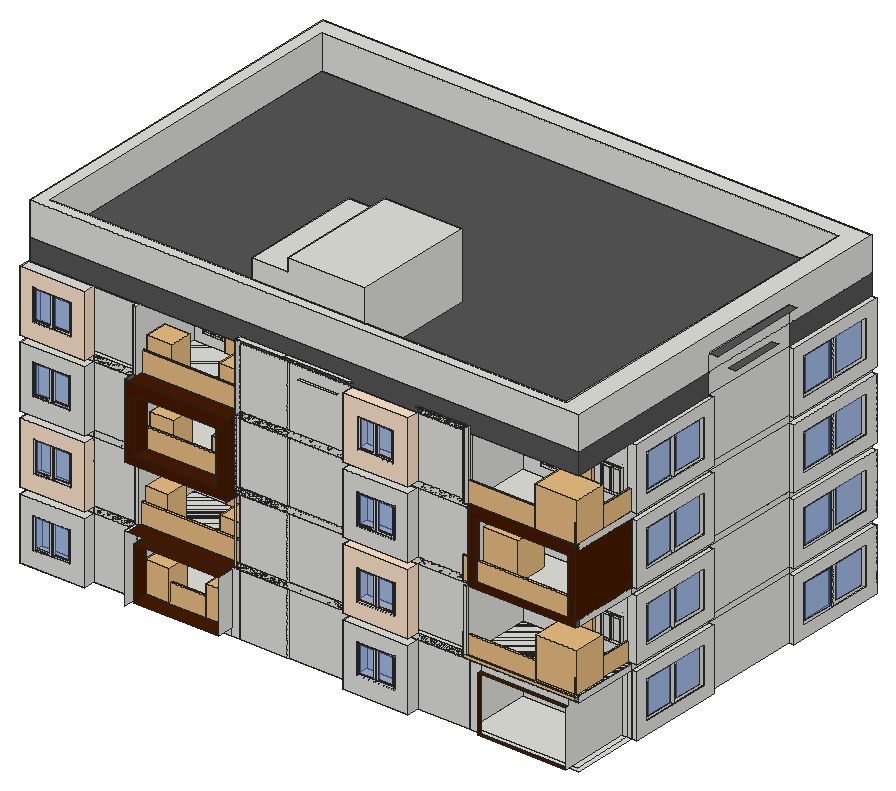
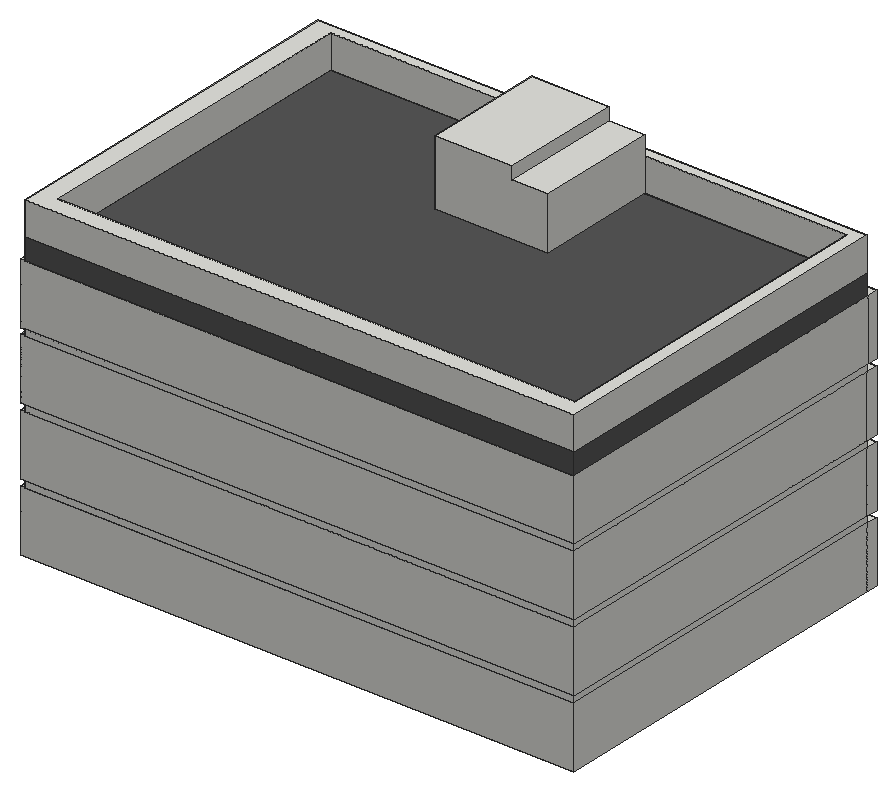
# SketchUp Ruby script. Lengths in inches.
U = 1.inch
M = Sketchup.active_model
def pt(a) = Geom::Point3d.new(a.map { |v| v * U })
def face(e, loops, mat)
  f = e.add_face(loops[0].map { |a| pt(a) })
  loops[1..].each { |l| e.add_face(l.map { |a| pt(a) }).erase! }
  f.material = f.back_material = mat if mat
  f
end
# faces: each face lists its corners as indices into pts; further lists are holes
def faces(e, pts, list, mat = nil) = list.each { |f| face(e, (f[0].is_a?(Array) ? f : [f]).map { |l| l.map { |i| pts[i] } }, mat) }
# xy, xz, yz: faces in a plane at the given z, y or x. An outline is a flat list of corners, or four numbers for a rectangle; further outlines are holes
def ring(l) = l.size == 4 ? [[l[0], l[1]], [l[2], l[1]], [l[2], l[3]], [l[0], l[3]]] : l.each_slice(2).to_a
def flat(e, list, mat, &to3) = list.each { |f| face(e, (f[0].is_a?(Array) ? f : [f]).map { |l| ring(l).map { |u, v| to3.(u, v) } }, mat) }
def xy(e, z, list, mat = nil) = flat(e, list, mat) { |x, y| [x, y, z] }
def xz(e, y, list, mat = nil) = flat(e, list, mat) { |x, z| [x, y, z] }
def yz(e, x, list, mat = nil) = flat(e, list, mat) { |y, z| [x, y, z] }
def lines(e, pts, list) = list.each { |a, b| e.add_line(pt(pts[a]), pt(pts[b])) }
# prism: a flat outline (further loops are holes) pulled along v
def prism(e, loops, v, mat = nil)
  f = face(e, loops, mat); d = Geom::Vector3d.new(v.map { |x| x * U })
  f.pushpull(f.normal.samedirection?(d) ? d.length : -d.length)
end
def box(e, o, s, mat = nil) = prism(e, [[o, [o[0] + s[0], o[1], o[2]], [o[0] + s[0], o[1] + s[1], o[2]], [o[0], o[1] + s[1], o[2]]]], [0, 0, s[2]], mat)
def at(x, y, z, deg = 0) = Geom::Transformation.translation(pt([x, y, z])) * Geom::Transformation.rotation(ORIGIN, Z_AXIS, deg.degrees)
def axes(o, x, y, z) = Geom::Transformation.new([*x, 0, *y, 0, *z, 0, *pt(o).to_a, 1])
def part(name) = M.definitions.add(name)
# library, detail: a bought-in or finely detailed component or shape, given as its bounding box
def library(name, o, s) = part(name).tap { |d| box(d.entities, o, s) }
def detail(e, o, s) = box(e.add_group.entities, o, s)
def put(e, d, t, mat = nil) = e.add_instance(d, t).tap { |i| i.material = mat if mat }
def group(e, t, mat = nil) = e.add_group.tap { |g| g.transformation = t; g.material = mat if mat }.entities
root = M.entities
M.materials.add("[Color C01]").color = [255, 229, 204]
M.materials.add("[Color C07]").color = [71, 27, 0]
M.materials.add("[Color M05]").color = [114, 114, 114]
M.materials.add("[Color M06]").color = [86, 86, 86]
M.materials.add("[Translucent Glass Blue]").color = [100, 149, 237]
M.materials["[Translucent Glass Blue]"].alpha = 0.5
c1 = library("porta 4",[0.2,-5.42,1.33],[46.55,4.72,83.21])
c2 = library("Glass balustrade section",[0,0,0],[60.75,3.875,44.35])
c3 = library("KentiaPalm",[-22.86,-14.31,0],[47.49,43.96,59.125])
c4 = part("Window")
xy(c4.entities,31.72,[[-0.78,88.6,2.72,128.1]])
xy(c4.entities,34.95,[[-0.78,91.53,0.84,106.59],[0.84,91.53,1.05,97.58],[1.05,91.53,1.42,106.59],[1.42,91.53,2.72,106.59],[0.84,97.58,1.05,98.18],
  [0.84,98.18,1.05,106.59]])
xy(c4.entities,35.27,[[-0.78,110.09,0.97,125.14],[1.05,110.09,2.72,125.14]])
xy(c4.entities,58.35,[[2.72,108.74,3.8,109.74]])
xy(c4.entities,77.8125,[[-0.78,110.09,2.72,125.14],[0.97,110.09,1.05,125.14]])
xy(c4.entities,77.93,[[-0.78,91.53,0.84,106.59],[1.05,91.53,1.42,106.59],[1.42,91.53,2.72,106.59]])
xy(c4.entities,80.72,[[-0.78,88.6,2.72,128.1]])
xz(c4.entities,88.6,[[-0.78,31.72,2.72,80.72]])
xz(c4.entities,91.53,[[-0.78,34.95,0.84,77.93],[1.05,34.95,1.42,77.93],[1.42,34.95,2.72,77.93]])
xz(c4.entities,106.59,[[-0.78,34.95,0.84,77.93],[0.84,34.95,1.05,77.93],[0.84,34.95,2.72,77.93]])
xz(c4.entities,108.74,[[3.8,54.35,4.22,54.6,4.22,59.47,2.72,59.97,2.72,58.35,3.8,58.35]])
xz(c4.entities,109.74,[[3.8,54.35,3.8,58.35,2.72,58.35,2.72,59.97,4.22,59.47,4.22,54.6]])
xz(c4.entities,110.09,[[-0.78,35.27,0.97,77.8125],[1.05,35.27,2.72,77.8125]])
xz(c4.entities,125.14,[[-0.78,35.27,0.97,77.8125],[0.97,35.27,1.05,80.72],[1.05,35.27,2.72,77.8125]])
xz(c4.entities,128.1,[[-0.78,31.72,2.72,80.72]])
yz(c4.entities,-0.78,[[[88.6,31.72,128.1,80.72],[91.53,34.95,106.59,77.93],[110.09,35.27,125.14,77.8125]]])
yz(c4.entities,0.84,[[91.53,34.95,106.59,77.93]])
yz(c4.entities,0.97,[[110.09,35.27,125.14,77.8125]])
yz(c4.entities,1.05,[[91.53,34.95,106.59,77.93],[110.09,35.27,125.14,77.8125]])
yz(c4.entities,1.42,[[91.53,34.95,106.59,77.93]])
yz(c4.entities,2.72,[[[88.6,31.72,108.35,80.72],[91.53,34.95,106.59,77.93]],[[108.35,31.72,128.1,80.72],[110.09,35.27,125.14,77.8125],[108.74,58.35,109.74,59.97]]])
yz(c4.entities,3.8,[[108.74,54.35,109.74,58.35]])
yz(c4.entities,4.22,[[108.74,54.6,109.74,59.47]])
p = [[4.22,108.74,54.6],[3.8,108.74,54.35],[3.8,109.74,54.35],[4.22,109.74,54.6],[2.72,109.74,59.97],[2.72,108.74,59.97],
  [4.22,108.74,59.47],[4.22,109.74,59.47],[-0.78,86.4,89.94],[-0.78,86.44,89.94],[15.22,130.69,89.94],[15.22,130.65,89.94],
  [-0.78,86.44,28.19],[-0.78,86.4,28.19],[7.72,130.69,89.94],[7.72,130.65,89.94]]
faces(c4.entities,p,[[0,1,2,3],[4,5,6,7]])
lines(c4.entities,p,[[8,9],[10,11],[12,13],[14,15]])
c5 = part("Janela aluminio")
xy(c5.entities,0,[[0,0,47.24,1.57],[23.62,1.57,47.24,2.76],[0,2.76,25.98,3.9375],[0,3.9375,47.24,5.91]])
xy(c5.entities,43.31,[[0,0,47.24,1.57],[23.62,1.57,47.24,2.76],[0,2.76,0,5.91,47.24,5.91,47.24,3.9375,25.98,3.9375,25.98,2.76],[25.98,2.76,47.24,3.9375]])
xz(c5.entities,1.57,[[0,0,23.62,0,23.62,41.34,21.26,41.34,21.26,1.97,1.97,1.97,1.97,41.34,23.62,41.34,23.62,43.31,0,43.31],[[23.62,0,47.24,43.31],[25.7,1.97,45.28,41.34]]])
xz(c5.entities,2.76,[[[0,0,23.62,43.31],[2.36,2.36,21.26,40.94]],[23.62,0,25.98,43.31]])
xz(c5.entities,2.76,[[2.36,2.36,21.26,40.94]],"[Translucent Glass Blue]")
xz(c5.entities,3.9375,[[25.98,0,25.98,2.36,44.88,2.36,44.88,40.94,25.98,40.94,25.98,43.31,47.24,43.31,47.24,0]])
xz(c5.entities,3.9375,[[25.98,2.36,44.88,40.94]],"[Translucent Glass Blue]")
yz(c5.entities,0,[[0,0,1.57,43.31],[2.76,0,5.91,43.31]])
yz(c5.entities,23.62,[[1.57,0,2.76,43.31]])
yz(c5.entities,25.98,[[2.76,0,3.9375,43.31]])
yz(c5.entities,47.24,[[0,0,1.57,43.31],[1.57,0,2.76,43.31],[3.9375,0,5.91,43.31]])
c6 = library("Round Planter with Plant",[-35.48,-39.77,0],[80.62,63.55,77.875])
xy(root,396,[[119.8125,172.4375,244.96,195.5625],[[119.8125,195.5625,327.85,195.5625,327.85,325.5625,528.67,325.5625,528.67,195.5625,974.8125,195.5625,974.8125,325.5625,1167.48,325.5625,1167.48,325.75,1186.5,325.75,1186.5,706.47,1196,706.47,1196,908.0625,119.8125,908.0625],[180.5,204.5625,180.5,894.25,1177.5,894.25,1177.5,334.5625,965.8125,334.5625,965.8125,204.5625,537.67,204.5625,537.67,334.5625,318.85,334.5625,318.85,204.5625]],[327.85,195.5625,528.67,204.5625],[974.8125,195.5625,1167.48,204.5625],[1167.48,195.5625,1167.48,204.5625,1177.5,204.5625,1177.5,325.5625,1186.5,325.5625,1186.5,195.5625],
  [180.5,204.5625,318.85,204.5625,318.85,334.5625,537.67,334.5625,537.67,204.5625,965.8125,204.5625,965.8125,334.5625,1177.5,334.5625,1177.5,894.25,180.5,894.25],[327.85,204.5625,528.67,325.5625],[974.8125,204.5625,1167.48,325.5625],[1167.48,204.5625,1177.5,325.5625],[1167.48,325.5625,1186.5,325.75],
  [1186.5,325.75,1196,513.49]])
xy(root,396,[[997.1,188.8125,1167.48,195.5625]],"[Color C07]")
xy(root,408.8125,[[345.85,165.375,511.9375,195.5625]],"[Color C07]")
xy(root,419.01,[[1188.1875,348.76,1196,490.48],[1188.1875,729.48,1196,885.06]])
xy(root,426.43,[[146.55,172.4375,215.84,191.375]])
xy(root,486.88,[[146.55,172.4375,215.84,191.375]])
xy(root,492.99,[[1188.1875,348.76,1196,490.48],[1188.1875,729.48,1196,885.06]])
xy(root,504.25,[[997.1,188.8125,1167.48,195.5625]],"[Color C07]")
xy(root,510.75,[[345.85,165.375,511.9375,195.5625]],"[Color C07]")
xy(root,516,[[119.8125,172.4375,244.96,195.5625],[[119.8125,195.5625,327.85,195.5625,327.85,325.5625,528.67,325.5625,528.67,195.5625,974.8125,195.5625,974.8125,325.5625,1167.48,325.5625,1167.48,325.75,1186.5,325.75,1186.5,706.47,1196,706.47,1196,908.0625,119.8125,908.0625],[180.5,204.5625,180.5,894.25,1177.5,894.25,1177.5,334.5625,965.8125,334.5625,965.8125,204.5625,537.67,204.5625,537.67,334.5625,318.85,334.5625,318.85,204.5625]],[1167.48,195.5625,1186.5,325.5625],[1167.48,325.5625,1186.5,325.75],[1186.5,325.75,1196,513.49]])
xy(root,528,[[327.85,165.375,334.29,191.75],[119.8125,172.4375,244.96,195.5625],[968.8125,188.3125,974.8125,191.25],[974.8125,188.8125,1178.19,195.5625],[1178.19,188.8125,1186.5,195.5625],
  [327.85,191.75,334.29,195.5625],[[119.8125,195.5625,334.29,195.5625,334.29,325.5625,528.67,325.5625,528.67,195.5625,974.8125,195.5625,974.8125,325.5625,1186.5,325.5625,1186.5,706.47,1196,706.47,1196,908.0625,119.8125,908.0625],[180.5,204.5625,180.5,894.25,1177.5,894.25,1177.5,334.5625,965.8125,334.5625,965.8125,204.5625,537.67,204.5625,537.67,334.5625,318.85,334.5625,318.85,204.5625]],[334.29,195.5625,528.67,204.5625],[974.8125,195.5625,1186.5,195.5625,1186.5,325.5625,1177.5,325.5625,1177.5,204.5625,974.8125,204.5625],[180.5,204.5625,318.85,204.5625,318.85,334.5625,537.67,334.5625,537.67,204.5625,965.8125,204.5625,965.8125,334.5625,1177.5,334.5625,1177.5,894.25,180.5,894.25],
  [334.29,204.5625,528.67,325.5625],[974.8125,204.5625,1177.5,325.5625],[1186.5,325.5625,1196,513.49]])
xy(root,528,[[334.29,165.375,528.5625,195.5625]],"[Color C07]")
xy(root,551.01,[[1188.1875,348.57,1196,490.48],[1188.1875,729.48,1196,885.06]])
xy(root,560.39,[[146.97,172.4375,217.8,187.75]])
xy(root,620.85,[[146.97,172.4375,217.8,187.75]])
xy(root,624.99,[[1188.1875,348.57,1196,490.48],[1188.1875,729.48,1196,885.06]])
xy(root,647.61,[[968.8125,188.3125,974.8125,191.25]])
xy(root,648,[[327.85,165.375,334.29,191.75],[119.8125,172.4375,244.96,195.5625],[974.8125,190.4375,1186.5,195.5625],[327.85,191.75,334.29,195.5625],[[119.8125,195.5625,334.29,195.5625,334.29,325.5625,528.67,325.5625,528.67,195.5625,974.8125,195.5625,974.8125,325.5625,1186.5,325.5625,1186.5,706.47,1196,706.47,1196,908.0625,119.8125,908.0625],[180.5,204.5625,180.5,894.25,1177.5,894.25,1177.5,334.5625,965.8125,334.5625,965.8125,204.5625,537.67,204.5625,537.67,334.5625,318.85,334.5625,318.85,204.5625]],
  [334.29,195.5625,528.67,325.5625],[974.8125,195.5625,1186.5,325.5625],[1186.5,325.5625,1196,513.49]])
xy(root,648,[[334.29,165.375,334.29,195.5625,528.67,195.5625,528.67,184.75,528.5625,184.75,528.5625,165.375]],"[Color C07]")
xy(root,660,[[119.8125,172.4375,244.96,195.5625],[992.25,190.4375,1169.54,195.5625],[[119.8125,195.5625,327.85,195.5625,327.85,325.5625,528.67,325.5625,528.67,195.5625,974.8125,195.5625,974.8125,325.5625,1169.54,325.5625,1169.54,325.625,1186.5,325.625,1186.5,706.47,1196,706.47,1196,908.0625,119.8125,908.0625],[180.5,204.5625,180.5,894.25,1177.5,894.25,1177.5,334.5625,965.8125,334.5625,965.8125,204.5625,537.67,204.5625,537.67,334.5625,318.85,334.5625,318.85,204.5625]],[327.85,195.5625,528.67,204.5625],[974.8125,195.5625,1169.54,204.5625],
  [1169.54,195.5625,1169.54,204.5625,1177.5,204.5625,1177.5,325.5625,1186.5,325.5625,1186.5,195.5625],[180.5,204.5625,318.85,204.5625,318.85,334.5625,537.67,334.5625,537.67,204.5625,965.8125,204.5625,965.8125,334.5625,1177.5,334.5625,1177.5,894.25,180.5,894.25],[327.85,204.5625,528.67,325.5625],[974.8125,204.5625,1169.54,325.5625],[1169.54,204.5625,1177.5,325.5625],
  [1169.54,325.5625,1186.5,325.625],[1186.5,325.625,1196,513.49]])
xy(root,664.5,[[347.98,165.375,506.15,195.5625]],"[Color C07]")
xy(root,683.01,[[1188.1875,348.63,1196,490.48],[1188.1875,729.48,1196,885.06]])
xy(root,694.08,[[145.28,172.4375,216.12,184.0625]])
xy(root,754.53,[[145.28,172.4375,216.12,184.0625]])
xy(root,756.99,[[1188.1875,348.63,1196,490.48],[1188.1875,729.48,1196,885.06]])
xy(root,769.01,[[347.98,165.375,506.15,195.5625]],"[Color C07]")
xy(root,770.375,[[992.25,190.4375,1169.54,195.5625]],"[Color C07]")
xy(root,780,[[119.8125,172.4375,244.96,195.5625],[[119.8125,195.5625,327.85,195.5625,327.85,325.5625,528.67,325.5625,528.67,195.5625,974.8125,195.5625,974.8125,325.5625,1169.54,325.5625,1169.54,325.625,1186.5,325.625,1186.5,706.47,1196,706.47,1196,908.0625,119.8125,908.0625],[180.5,204.5625,180.5,894.25,1177.5,894.25,1177.5,334.5625,965.8125,334.5625,965.8125,204.5625,537.67,204.5625,537.67,334.5625,318.85,334.5625,318.85,204.5625]],[1169.54,195.5625,1186.5,325.5625],[1169.54,325.5625,1186.5,325.625],[1186.5,325.625,1196,513.49]])
xy(root,792,[[119.8125,172.4375,244.96,193.5625],[327.85,184.75,335.54,195.5625],[974.19,185.85,968.19,186.67,968.8125,191.25,974.8125,190.4375],[974.8125,190.4375,1186.5,190.4375,1186.5,325.5625,1177.5,325.5625,1177.5,204.5625,974.8125,204.5625],[[119.8125,193.5625,244.96,193.5625,244.96,195.5625,335.54,195.5625,335.54,325.5625,528.67,325.5625,528.67,195.5625,974.8125,195.5625,974.8125,325.5625,1186.5,325.5625,1186.5,706.47,1196,706.47,1196,908.0625,119.8125,908.0625],[180.5,204.5625,180.5,894.25,1177.5,894.25,1177.5,334.5625,965.8125,334.5625,965.8125,204.5625,537.67,204.5625,537.67,334.5625,318.85,334.5625,318.85,204.5625]],
  [335.54,195.5625,528.67,204.5625],[180.5,204.5625,318.85,204.5625,318.85,334.5625,537.67,334.5625,537.67,204.5625,965.8125,204.5625,965.8125,334.5625,1177.5,334.5625,1177.5,894.25,180.5,894.25],[335.54,204.5625,528.67,325.5625],[974.8125,204.5625,1177.5,325.5625],[1186.5,325.5625,1196,513.49]])
xy(root,792,[[335.54,165.375,528.5625,165.375,528.5625,184.75,528.67,184.75,528.67,195.5625,335.54,195.5625]],"[Color C07]")
xy(root,792,[[327.85,165.375,335.54,184.75]],"[Color M06]")
xy(root,815.01,[[1188.1875,348.57,1196,490.48],[1188.1875,729.48,1196,885.06]])
xy(root,823.75,[[147.61,172.4375,217.16,184.125]])
xy(root,884.2,[[147.61,172.4375,217.16,184.125]])
xy(root,888.99,[[1188.1875,348.57,1196,490.48],[1188.1875,729.48,1196,885.06]])
xy(root,893.47,[[647.73,187.0625,723.37,190.9375]])
xy(root,912,[[119.8125,172.4375,244.96,193.5625],[[327.85,184.75,335.54,184.75,335.54,325.5625,528.67,325.5625,528.67,195.5625,974.8125,195.5625,974.8125,325.5625,1196,325.5625,1196,513.49,1186.5,513.49,1186.5,706.47,1196,706.47,1196,908.0625,119.8125,908.0625,119.8125,193.5625,325.71,193.5625,325.71,195.5625,327.85,195.5625],[180.5,204.5625,180.5,894.25,1177.5,894.25,1177.5,334.5625,965.8125,334.5625,965.8125,204.5625,537.67,204.5625,537.67,334.5625,318.85,334.5625,318.85,204.5625]]])
xy(root,924,[[528.67,184.75,620.44,195.5625],[974.19,185.85,974.8125,190.4375,968.8125,191.25,968.19,186.67],[622.95,187.0625,747.02,195.5625],[968.8125,191.25,975.125,193.6875],[873.5,193.6875,974.8125,195.5625]])
xy(root,924,[[528.5625,182.3125,534.875,184.75],[873.5,191.25,879.8125,193.6875],[881.6875,191.25,888,193.6875],[889.4375,191.25,895.75,193.6875],[897.25,191.25,903.5625,193.6875],
  [904.8125,191.25,911.125,193.6875],[912.5,191.25,918.8125,193.6875],[920.25,191.25,926.5625,193.6875],[928.4375,191.25,934.75,193.6875],[936.8125,191.25,943.125,193.6875],
  [944.8125,191.25,951.125,193.6875],[952.8125,191.25,959.125,193.6875],[961.375,191.25,967.6875,193.6875]],"[Color M05]")
xy(root,941.41,[[1189.6875,557.39,1202.5625,662.57]],"[Color M06]")
xy(root,952.5,[[[119.8125,195.5625,1186.5,908.0625],[144.17,213.9,1148.29,875.62]]])
xy(root,985.3125,[[1186.5,513.49,1202.5625,706.47]],"[Color M06]")
xy(root,1017.9375,[[[119.8125,195.5625,1186.5,908.0625],[144.17,213.9,1148.29,875.62]]])
xy(root,1054.86,[[536.28,213.9,606.15,450.15]])
xy(root,1079.25,[[606.15,213.9,756.53,450.15]])
xz(root,165.375,[[[327.85,648,528.5625,792],[347.98,664.5,506.15,769.01]]],"[Color C07]")
xz(root,172.4375,[[[119.8125,396,244.96,516],[146.55,426.43,215.84,486.88]],[[119.8125,660,244.96,780],[145.28,694.08,216.12,754.53]]])
xz(root,172.4375,[[[119.8125,528,244.96,648],[146.97,560.39,217.8,620.85]],[[119.8125,792,244.96,912],[147.61,823.75,217.16,884.2]]],"[Color C01]")
xz(root,184.0625,[[145.28,694.08,216.12,754.53]])
xz(root,184.125,[[147.61,823.75,217.16,884.2]])
xz(root,184.75,[[327.85,792,335.54,912]])
xz(root,184.75,[[528.5625,648,528.67,792]],"[Color M06]")
xz(root,187.75,[[146.97,560.39,217.8,620.85]])
xz(root,188.3125,[[968.8125,528,974.8125,647.61]])
xz(root,190.4375,[[[974.8125,648,1186.5,792],[992.25,660,1169.54,770.375]]],"[Color C07]")
xz(root,191.375,[[146.55,426.43,215.84,486.88]])
xz(root,191.75,[[327.85,528,334.29,648]])
xz(root,193.5625,[[119.8125,792,244.96,912]])
xz(root,195.5625,[[119.8125,396,244.96,516],[244.96,396,325.71,516],[325.71,396,327.85,516],[327.85,396,327.85,528,528.5625,528,528.5625,396,511.9375,396,511.9375,510.75,345.85,510.75,345.85,396],[345.85,396,511.9375,408.8125],
  [528.67,396,620.44,516],[620.44,396,622.95,516],[622.95,396,747.02,516],[747.02,396,873.5,516],[873.5,396,974.8125,516],
  [974.8125,396,997.1,516],[997.1,504.25,997.1,516,974.8125,516,974.8125,528,1186.5,528,1186.5,516,1167.48,516,1167.48,504.25],[244.96,516,325.71,528],[528.67,516,620.44,528],[622.95,516,747.02,528],
  [873.5,516,974.8125,528],[119.8125,528,244.96,648],[244.96,528,325.71,648],[325.71,528,327.85,648],[528.67,528,620.44,648],
  [620.44,528,622.95,648],[622.95,528,747.02,648],[747.02,528,873.5,648],[244.96,648,325.71,660],[327.85,648,528.67,660],
  [528.67,648,620.44,660],[622.95,648,747.02,660],[873.5,648,974.8125,660],[974.8125,648,1186.5,660],[119.8125,660,244.96,780],
  [244.96,660,325.71,780],[325.71,660,327.85,780],[327.85,660,347.98,780.01],[518.65,660,518.65,664.5,506.15,664.5,506.15,769.01,347.98,769.01,347.98,780.01,327.85,780.01,327.85,792,528.67,792,528.67,660],[347.98,660,518.65,664.5],
  [528.67,660,620.44,780],[620.44,660,622.95,780],[622.95,660,747.02,780],[747.02,660,873.5,780],[873.5,660,974.8125,780],
  [992.25,770.375,1169.54,780],[244.96,780,325.71,792],[528.67,780,620.44,792],[622.95,780,747.02,792],[873.5,780,974.8125,792],
  [325.71,792,327.85,912],[528.67,792,620.44,912],[620.44,792,622.95,912],[622.95,792,747.02,912],[747.02,792,873.5,912],
  [873.5,792,974.8125,912],[528.67,912,620.44,924],[622.95,912,747.02,924],[873.5,912,974.8125,924],[119.8125,952.5,1186.5,1017.9375]])
xz(root,204.5625,[[180.5,396,318.85,516],[537.67,396,965.8125,516],[180.5,528,318.85,648],[537.67,528,965.8125,648],[180.5,660,318.85,780],
  [537.67,660,965.8125,780],[180.5,792,318.85,912],[537.67,792,965.8125,912]])
xz(root,213.9,[[144.17,952.5,536.28,1017.9375],[536.28,952.5,756.53,1017.9375],[756.53,952.5,1148.29,1017.9375],[536.28,1017.9375,536.28,1054.86,606.15,1054.86,606.15,1079.25,756.53,1079.25,756.53,1017.9375]])
xz(root,325.5625,[[327.85,396,528.67,516],[974.8125,396,1177.5,516],[1177.5,396,1186.5,516],[334.29,528,528.67,648],[974.8125,528,1177.5,648],
  [1177.5,528,1196,648],[327.85,660,528.67,780],[974.8125,660,1177.5,780],[1177.5,660,1186.5,780],[335.54,792,528.67,912],
  [974.8125,792,1177.5,912],[1177.5,792,1196,912]])
xz(root,325.625,[[1169.54,660,1186.5,780],[1186.5,660,1196,780]])
xz(root,325.75,[[1167.48,396,1186.5,516],[1186.5,396,1196,516]])
xz(root,334.5625,[[318.85,396,537.67,516],[965.8125,396,1177.5,516],[318.85,528,537.67,648],[965.8125,528,1177.5,648],[318.85,660,537.67,780],
  [965.8125,660,1177.5,780],[318.85,792,537.67,912],[965.8125,792,1177.5,912]])
xz(root,348.57,[[1188.1875,551.01,1196,624.99],[1188.1875,815.01,1196,888.99]])
xz(root,348.63,[[1188.1875,683.01,1196,756.99]])
xz(root,348.76,[[1188.1875,419.01,1196,492.99]])
xz(root,450.15,[[536.28,952.5,756.53,952.5,756.53,1079.25,606.15,1079.25,606.15,1054.86,536.28,1054.86]])
xz(root,490.48,[[1188.1875,419.01,1196,492.99],[1188.1875,551.01,1196,624.99],[1188.1875,683.01,1196,756.99],[1188.1875,815.01,1196,888.99]])
xz(root,513.49,[[1186.5,396,1196,516],[1186.5,528,1196,648],[1186.5,660,1196,780],[1186.5,792,1196,912]])
xz(root,706.47,[[1186.5,396,1196,516],[1186.5,528,1196,648],[1186.5,660,1196,780],[1186.5,792,1196,912]])
xz(root,729.48,[[1188.1875,419.01,1196,492.99],[1188.1875,551.01,1196,624.99],[1188.1875,683.01,1196,756.99],[1188.1875,815.01,1196,888.99]])
xz(root,875.62,[[144.17,952.5,1148.29,1017.9375]])
xz(root,885.06,[[1188.1875,419.01,1196,492.99],[1188.1875,551.01,1196,624.99],[1188.1875,683.01,1196,756.99],[1188.1875,815.01,1196,888.99]])
xz(root,894.25,[[180.5,396,1177.5,516],[180.5,528,1177.5,648],[180.5,660,1177.5,780],[180.5,792,1177.5,912]])
xz(root,908.0625,[[119.8125,396,1196,516],[119.8125,528,1196,648],[119.8125,660,1196,780],[119.8125,792,1196,912],[119.8125,952.5,1186.5,1017.9375]])
yz(root,119.8125,[[172.4375,396,195.5625,516],[195.5625,396,908.0625,516],[172.4375,528,195.5625,648],[195.5625,528,908.0625,648],[172.4375,660,195.5625,780],
  [195.5625,660,908.0625,780],[172.4375,792,193.5625,912],[193.5625,792,908.0625,912],[195.5625,952.5,908.0625,1017.9375]])
yz(root,144.17,[[213.9,952.5,875.62,1017.9375]])
yz(root,145.28,[[172.4375,694.08,184.0625,754.53]])
yz(root,146.55,[[172.4375,426.43,191.375,486.88]])
yz(root,146.97,[[172.4375,560.39,187.75,620.85]])
yz(root,147.61,[[172.4375,823.75,184.125,884.2]])
yz(root,180.5,[[204.5625,396,894.25,516],[204.5625,528,894.25,648],[204.5625,660,894.25,780],[204.5625,792,894.25,912]])
yz(root,215.84,[[172.4375,426.43,191.375,486.88]])
yz(root,216.12,[[172.4375,694.08,184.0625,754.53]])
yz(root,217.16,[[172.4375,823.75,184.125,884.2]])
yz(root,217.8,[[172.4375,560.39,187.75,620.85]])
yz(root,244.96,[[172.4375,396,193.5625,516],[193.5625,396,195.5625,516],[193.5625,516,195.5625,528],[193.5625,528,195.5625,648],[193.5625,648,195.5625,660],
  [172.4375,660,193.5625,780],[193.5625,660,195.5625,780],[193.5625,780,195.5625,792]])
yz(root,244.96,[[172.4375,528,193.5625,648],[172.4375,792,193.5625,912]],"[Color C01]")
yz(root,318.85,[[204.5625,396,334.5625,516],[204.5625,528,334.5625,648],[204.5625,660,334.5625,780],[204.5625,792,334.5625,912]])
yz(root,327.85,[[165.375,396,195.5625,528],[195.5625,396,204.5625,516],[204.5625,396,325.5625,516],[191.75,528,195.5625,648],[165.375,648,195.5625,780.01],
  [195.5625,660,204.5625,780],[204.5625,660,325.5625,780],[165.375,780.01,195.5625,792],[184.75,792,195.5625,912]])
yz(root,334.29,[[191.75,528,325.5625,648]])
yz(root,335.54,[[184.75,792,325.5625,912]])
yz(root,345.85,[[165.375,408.8125,195.5625,510.75]],"[Color C07]")
yz(root,347.98,[[165.375,664.5,195.5625,769.01]],"[Color C07]")
yz(root,506.15,[[165.375,664.5,195.5625,769.01]])
yz(root,511.9375,[[165.375,408.8125,195.5625,510.75]])
yz(root,528.5625,[[182.3125,528,184.75,648],[182.3125,648,184.75,792],[182.3125,792,184.75,924]])
yz(root,528.5625,[[165.375,648,182.3125,792]],"[Color C07]")
yz(root,528.67,[[195.5625,396,204.5625,516],[204.5625,396,325.5625,516],[195.5625,528,204.5625,648],[204.5625,528,325.5625,648],[195.5625,660,204.5625,780],
  [204.5625,660,325.5625,780],[184.75,792,195.5625,924],[195.5625,792,204.5625,912],[204.5625,792,325.5625,912]])
yz(root,536.28,[[213.9,952.5,450.15,1054.86]])
yz(root,537.67,[[204.5625,396,334.5625,516],[204.5625,528,334.5625,648],[204.5625,660,334.5625,780],[204.5625,792,334.5625,912]])
yz(root,606.15,[[213.9,1054.86,450.15,1079.25]])
yz(root,756.53,[[213.9,952.5,450.15,1079.25]])
yz(root,965.8125,[[204.5625,396,334.5625,516],[204.5625,528,334.5625,648],[204.5625,660,334.5625,780],[204.5625,792,334.5625,912]])
yz(root,974.8125,[[195.5625,396,204.5625,516],[204.5625,396,325.5625,516],[188.3125,528,191.25,647.61],[193.6875,528,325.5625,648],[190.4375,648,193.6875,660],
  [193.6875,648,195.5625,660],[190.4375,660,193.6875,792],[193.6875,660,195.5625,792],[195.5625,660,204.5625,780],[204.5625,660,325.5625,780],
  [193.6875,792,195.5625,924],[195.5625,792,204.5625,912],[204.5625,792,325.5625,912]])
yz(root,992.25,[[190.4375,660,195.5625,770.375]],"[Color C07]")
yz(root,997.1,[[188.8125,396,195.5625,504.25]],"[Color C07]")
yz(root,1148.29,[[213.9,952.5,875.62,1017.9375]])
yz(root,1167.48,[[188.8125,396,188.8125,504.25,195.5625,504.25,195.5625,516,325.75,516,325.75,396]])
yz(root,1169.54,[[190.4375,660,190.4375,770.375,195.5625,770.375,195.5625,780,325.625,780,325.625,660]])
yz(root,1177.5,[[334.5625,396,894.25,516],[334.5625,528,894.25,648],[334.5625,660,894.25,780],[334.5625,792,894.25,912]])
yz(root,1186.5,[[325.5625,396,325.75,516],[513.49,396,706.47,516],[325.3125,516,513.49,516,513.49,528,195.5625,528,195.5625,527.5,325.3125,527.5],[513.49,516,706.47,528],[513.49,528,706.47,648],
  [325.5625,648,513.49,660],[513.49,648,706.47,660],[325.5625,660,325.625,780],[513.49,660,706.47,780],[513.49,780,706.47,792],
  [513.49,792,706.47,912],[513.49,912,706.47,952.5],[195.5625,952.5,513.49,952.5,513.49,985.3125,706.47,985.3125,706.47,952.5,908.0625,952.5,908.0625,1017.9375,195.5625,1017.9375],[513.49,952.5,706.47,985.3125]])
yz(root,1186.5,[[195.5625,516,325.3125,527.5],[195.5625,648,325.5625,660],[190.4375,660,325.5625,660,325.5625,780,195.5625,780,195.5625,792,190.4375,792],[195.5625,780,513.49,792]],"[Color C07]")
yz(root,1186.5,[[190.4375,648,195.5625,660]],"[Color M06]")
yz(root,1188.1875,[[348.76,419.01,490.48,492.99],[729.48,419.01,885.06,492.99],[348.57,551.01,490.48,624.99],[729.48,551.01,885.06,624.99],[348.63,683.01,490.48,756.99],
  [729.48,683.01,885.06,756.99],[348.57,815.01,490.48,888.99],[729.48,815.01,885.06,888.99]])
yz(root,1196,[[[325.75,396,513.49,516],[348.76,419.01,490.48,492.99]],[[706.47,396,908.0625,516],[729.48,419.01,885.06,492.99]],[[325.5625,528,513.49,648],[348.57,551.01,490.48,624.99]],[[706.47,528,908.0625,648],[729.48,551.01,885.06,624.99]],[[325.625,660,513.49,780],[348.63,683.01,490.48,756.99]],
  [[706.47,660,908.0625,780],[729.48,683.01,885.06,756.99]],[[325.5625,792,513.49,912],[348.57,815.01,490.48,888.99]],[[706.47,792,908.0625,912],[729.48,815.01,885.06,888.99]]])
p = [[968.19,186.67,792],[974.19,185.85,792],[974.19,185.85,924],[968.19,186.67,924],[974.8125,190.4375,792],[974.8125,190.4375,924],
  [968.8125,191.25,924],[968.8125,191.25,792]]
faces(root,p,[[0,1,2,3],[4,5,2,1],[6,7,0,3],[4,7,6,5]])
g1 = group(root,at(747.02,195.5625,396))
xy(g1,0,[[0,-23.125,126.48,0]])
xy(g1,36.18,[[28.18,-23.125,100.24,0]])
xy(g1,92.01,[[28.18,-23.125,100.24,0]])
xy(g1,120,[[0,-23.125,126.48,0]])
xz(g1,-23.125,[[[0,0,126.48,120],[28.18,36.18,100.24,92.01]]])
xz(g1,0,[[[0,0,126.48,120],[28.18,36.18,100.24,92.01]],[28.18,36.18,100.24,92.01]])
yz(g1,0,[[-23.125,0,0,120]])
yz(g1,28.18,[[-23.125,36.18,0,92.01]])
yz(g1,100.24,[[-23.125,36.18,0,92.01]])
yz(g1,126.48,[[-23.125,0,0,120]])
put(root,c1,at(1067.5625,325.5625,397.87))
put(root,c1,at(400.125,325.5625,397.87))
put(root,c2,axes([320.66,197.45,402.0625],[3.42226,0,0],[0,1,0],[0,0,1]))
put(root,c3,at(485.74,209.71,410.73))
put(root,c3,at(366.31,209.71,410.73))
put(root,c4,at(1249.11,314.34,388.99,90))
put(root,c4,at(1131.67,314.34,388.99,90))
put(root,c4,at(592.54,314.34,388.99,90))
put(root,c4,at(475.11,314.34,388.99,90))
put(root,c5,axes([1188.68,490.48,419.01],[0,-2.99951,0],[1.24,0,0],[0,0,1.70845]))
put(root,c5,axes([1188.68,885.06,419.01],[0,-3.30143,0],[1.24,0,0],[0,0,1.70845]))
put(root,c5,axes([143.77,172.4375,426.43],[1.5254,0,0],[0,1,0],[0,0,1.39595]))
put(root,c5,axes([775.19,171.02,430.12],[1.5254,0,0],[0,1.24,0],[0,0,1.33678]))
g2 = group(root,at(171.4375,908.0625,516))
box(g2,[-51.625,-712.5,0],[1066.6875,712.5,12])
put(root,c2,axes([964.11,192.375,519.19],[3.60079,0,0],[0,1,0],[0,0,1]))
put(root,c2,axes([1174.375,333.34,522.41],[0,-2.16255,0],[1,0,0],[0,0,0.89]))
put(root,c2,axes([320.66,197.45,522.6875],[3.42226,0,0],[0,1,0],[0,0,1]))
g3 = group(root,at(747.02,195.5625,528),"[Color C01]")
xy(g3,0,[[0,-23.125,126.48,0]])
xy(g3,32.93,[[28.18,-23.125,100.24,0]])
xy(g3,88.51,[[28.18,-23.125,100.24,0]])
xy(g3,120,[[0,-23.125,126.48,0]])
xz(g3,-23.125,[[[0,0,126.48,120],[28.18,32.93,100.24,88.51]]])
xz(g3,0,[[[0,0,126.48,120],[28.18,32.93,100.24,88.51]],[28.18,32.93,100.24,88.51]])
yz(g3,0,[[-23.125,0,0,120]])
yz(g3,28.18,[[-23.125,32.93,0,88.51]])
yz(g3,100.24,[[-23.125,32.93,0,88.51]])
yz(g3,126.48,[[-23.125,0,0,120]])
put(root,c3,at(354.76,221.74,530.3))
put(root,c3,at(503.08,221.74,530.3))
put(root,c1,at(1067.5625,325.5625,529.87))
put(root,c1,at(400.125,325.5625,529.87))
put(root,c6,at(1142.5,230.63,531.4))
put(root,c4,at(1139.99,321.92,522.24,90))
put(root,c4,at(1257.43,321.92,522.24,90))
put(root,c4,at(600.86,321.92,522.24,90))
put(root,c4,at(483.43,321.92,522.24,90))
put(root,c5,axes([1188.68,885.06,551.01],[0,-3.30143,0],[1.24,0,0],[0,0,1.70845]))
put(root,c5,axes([1188.68,490.48,551.01],[0,-2.99951,0],[1.24,0,0],[0,0,1.70845]))
put(root,c5,axes([775.19,171.02,558.62],[1.5254,0,0],[0,1.24,0],[0,0,1.33678]))
put(root,c5,axes([145.74,172.4375,560.39],[1.5254,0,0],[0,1,0],[0,0,1.39595]))
g4 = group(root,at(171.4375,908.0625,648))
box(g4,[-51.625,-712.5,0],[1066.6875,712.5,12])
put(root,c2,axes([964.11,192.375,653.38],[3.60079,0,0],[0,1,0],[0,0,1]))
put(root,c2,axes([320.66,197.45,656.5],[3.42226,0,0],[0,1,0],[0,0,1]))
put(root,c6,at(997.6,266.72,656.78))
g5 = group(root,at(747.02,195.5625,660))
xy(g5,0,[[0,-23.125,126.48,0]])
xy(g5,30.99,[[28.18,-23.125,100.24,0]])
xy(g5,89.26,[[28.18,-23.125,100.24,0]])
xy(g5,120,[[0,-23.125,126.48,0]])
xz(g5,-23.125,[[[0,0,126.48,120],[28.18,30.99,100.24,89.26]]])
xz(g5,0,[[[0,0,126.48,120],[28.18,30.99,100.24,89.26]],[28.18,30.99,100.24,89.26]])
yz(g5,0,[[-23.125,0,0,120]])
yz(g5,28.18,[[-23.125,30.99,0,89.26]])
yz(g5,100.24,[[-23.125,30.99,0,89.26]])
yz(g5,126.48,[[-23.125,0,0,120]])
put(root,c1,at(1067.5625,325.5625,661.32))
put(root,c1,at(400.125,325.5625,661.32))
put(root,c3,at(487.08,221.74,662.99))
put(root,c3,at(366.08,221.74,662.99))
put(root,c4,at(1139.99,314.34,653.8,90))
put(root,c4,at(1257.43,314.34,653.8,90))
put(root,c4,at(483.43,314.34,653.8,90))
put(root,c4,at(600.86,314.34,653.8,90))
put(root,c5,axes([1188.68,885.06,683.01],[0,-3.30143,0],[1.24,0,0],[0,0,1.70845]))
put(root,c5,axes([1188.68,490.48,683.01],[0,-2.99951,0],[1.24,0,0],[0,0,1.70845]))
put(root,c5,axes([775.19,171.02,691.37],[1.5254,0,0],[0,1.24,0],[0,0,1.33678]))
put(root,c5,axes([144.05,172.4375,694.08],[1.5254,0,0],[0,1,0],[0,0,1.39595]))
g6 = group(root,at(171.4375,908.0625,780))
box(g6,[-51.625,-712.5,0],[1066.6875,712.5,12])
put(root,c2,axes([320.66,197.45,786.3125],[3.42226,0,0],[0,1,0],[0,0,1]))
put(root,c2,axes([964.11,192.375,787.01],[3.60079,0,0],[0,1,0],[0,0,1]))
g7 = group(root,at(747.02,195.5625,792),"[Color C01]")
xy(g7,0,[[0,-23.125,126.48,0]])
xy(g7,31.93,[[28.18,-23.125,97.24,0]])
xy(g7,88.76,[[28.18,-23.125,97.24,0]])
xy(g7,120,[[0,-23.125,126.48,0]])
xz(g7,-23.125,[[[0,0,126.48,120],[28.18,31.93,97.24,88.76]]])
xz(g7,0,[[[0,0,126.48,120],[28.18,31.93,97.24,88.76]],[28.18,31.93,97.24,88.76]])
yz(g7,0,[[-23.125,0,0,120]])
yz(g7,28.18,[[-23.125,31.93,0,88.76]])
yz(g7,97.24,[[-23.125,31.93,0,88.76]])
yz(g7,126.48,[[-23.125,0,0,120]])
put(root,c2,axes([1181.375,325.5625,792],[0,-2.16255,0],[1,0,0],[0,0,0.89]))
put(root,c6,at(1140.63,231.375,792.17))
put(root,c1,at(1065.625,325.5625,792.89))
put(root,c1,at(398.1875,325.5625,792.89))
put(root,c3,at(360.86,221.74,794.58))
put(root,c3,at(501.49,221.74,794.58))
put(root,c4,at(1139.99,322.78,780.49,90))
put(root,c4,at(1257.43,322.78,780.49,90))
put(root,c4,at(483.43,322.78,780.49,90))
put(root,c4,at(600.86,322.78,780.49,90))
put(root,c5,axes([1188.68,885.06,815.01],[0,-3.30143,0],[1.24,0,0],[0,0,1.70845]))
put(root,c5,axes([1188.68,490.48,815.01],[0,-2.99951,0],[1.24,0,0],[0,0,1.70845]))
put(root,c5,axes([775.19,172.4375,822.87],[1.46184,0,0],[0,1.24,0],[0,0,1.33678]))
put(root,c5,axes([145.09,172.4375,823.75],[1.5254,0,0],[0,1,0],[0,0,1.39595]))
g8 = group(root,at(171.4375,908.0625,912),"[Color M06]")
box(g8,[-51.625,-712.5,0],[1066.6875,712.5,40.5])
